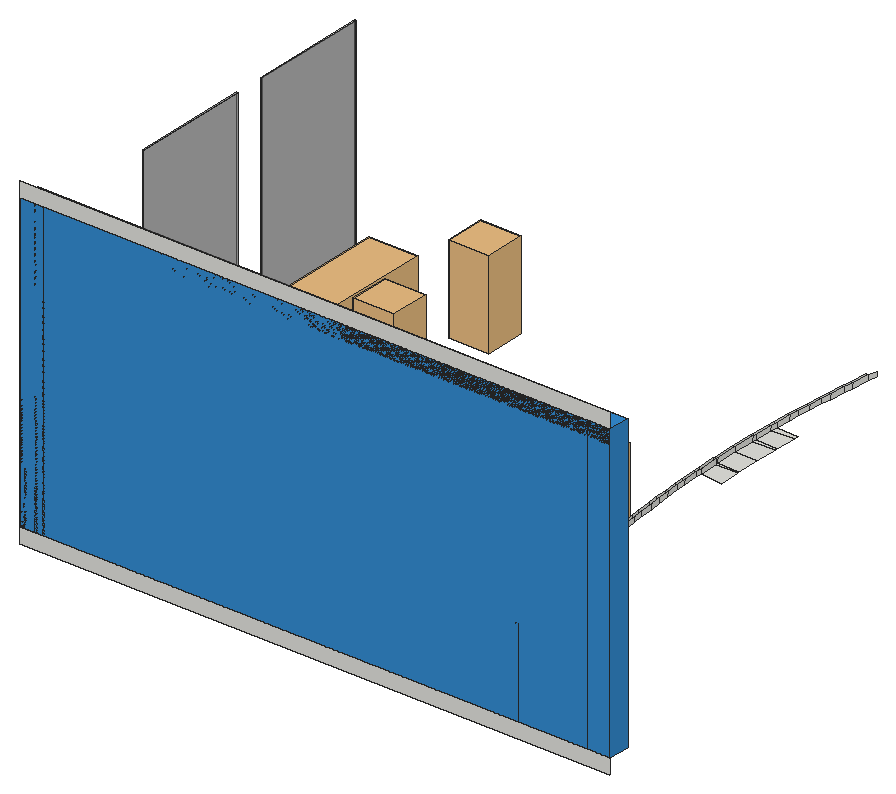
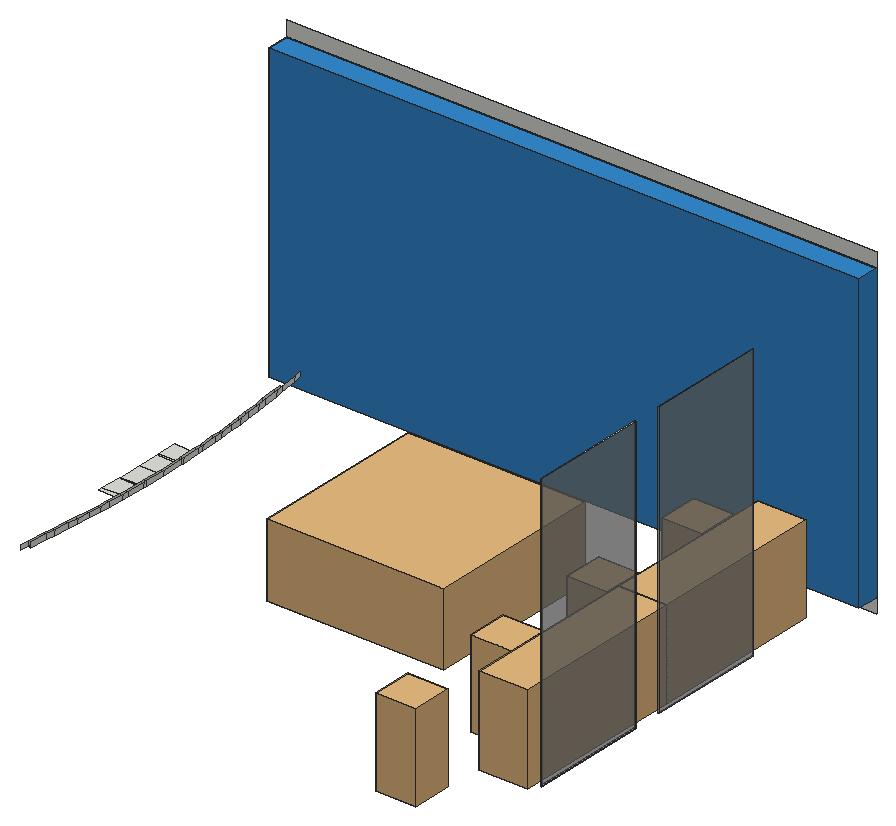
# SketchUp Ruby script. Lengths in inches.
U = 1.inch
M = Sketchup.active_model
def pt(a) = Geom::Point3d.new(a.map { |v| v * U })
def face(e, loops, mat)
  f = e.add_face(loops[0].map { |a| pt(a) })
  loops[1..].each { |l| e.add_face(l.map { |a| pt(a) }).erase! }
  f.material = f.back_material = mat if mat
  f
end
# faces: each face lists its corners as indices into pts; further lists are holes
def faces(e, pts, list, mat = nil) = list.each { |f| face(e, (f[0].is_a?(Array) ? f : [f]).map { |l| l.map { |i| pts[i] } }, mat) }
# xy, xz, yz: faces in a plane at the given z, y or x. An outline is a flat list of corners, or four numbers for a rectangle; further outlines are holes
def ring(l) = l.size == 4 ? [[l[0], l[1]], [l[2], l[1]], [l[2], l[3]], [l[0], l[3]]] : l.each_slice(2).to_a
def flat(e, list, mat, &to3) = list.each { |f| face(e, (f[0].is_a?(Array) ? f : [f]).map { |l| ring(l).map { |u, v| to3.(u, v) } }, mat) }
def xy(e, z, list, mat = nil) = flat(e, list, mat) { |x, y| [x, y, z] }
def xz(e, y, list, mat = nil) = flat(e, list, mat) { |x, z| [x, y, z] }
def yz(e, x, list, mat = nil) = flat(e, list, mat) { |y, z| [x, y, z] }
def lines(e, pts, list) = list.each { |a, b| e.add_line(pt(pts[a]), pt(pts[b])) }
# prism: a flat outline (further loops are holes) pulled along v
def prism(e, loops, v, mat = nil)
  f = face(e, loops, mat); d = Geom::Vector3d.new(v.map { |x| x * U })
  f.pushpull(f.normal.samedirection?(d) ? d.length : -d.length)
end
def box(e, o, s, mat = nil) = prism(e, [[o, [o[0] + s[0], o[1], o[2]], [o[0] + s[0], o[1] + s[1], o[2]], [o[0], o[1] + s[1], o[2]]]], [0, 0, s[2]], mat)
def at(x, y, z, deg = 0) = Geom::Transformation.translation(pt([x, y, z])) * Geom::Transformation.rotation(ORIGIN, Z_AXIS, deg.degrees)
def axes(o, x, y, z) = Geom::Transformation.new([*x, 0, *y, 0, *z, 0, *pt(o).to_a, 1])
def part(name) = M.definitions.add(name)
# library, detail: a bought-in or finely detailed component or shape, given as its bounding box
def library(name, o, s) = part(name).tap { |d| box(d.entities, o, s) }
def detail(e, o, s) = box(e.add_group.entities, o, s)
def put(e, d, t, mat = nil) = e.add_instance(d, t).tap { |i| i.material = mat if mat }
def group(e, t, mat = nil) = e.add_group.tap { |g| g.transformation = t; g.material = mat if mat }.entities
root = M.entities
M.materials.add("[Color I07]").color = [53, 140, 209]
M.materials.add("[Translucent Glass Gray]").color = [128, 128, 128]
M.materials["[Translucent Glass Gray]"].alpha = 0.5
M.materials.add("[Wood Veneer 02]").color = [190, 128, 91]
c1 = library("Edge Console",[-35.43,-9.84,0],[70.86,19.68,29.53])
c2 = library("Group\#15",[-0.03,0,0],[16.43,16.29,39.54])
c3 = library("MARBLE DINING TABLE",[-16.8,-22.21,-0.08],[92.52,94.06,29.61])
c4 = part("Group45\#1")
xz(c4.entities,3.52,[[223.67,42,224.7,44]])
c5 = part("Group49\#1")
xz(c5.entities,3.52,[[21.9,6,30.9,126]],"[Color I07]")
c6 = part("Group53\#1")
xz(c6.entities,3.52,[[21.9,0,261.9,6]])
c7 = part("Group593\#1")
xz(c7.entities,3.52,[[21.9,126.1875,261.9,132.1875]])
c8 = part("Group595\#1")
xz(c8.entities,3.52,[[21.9,120.1875,261.9,126.1875]],"[Color I07]")
c9 = part("Group663\#1")
xz(c9.entities,3.52,[[21.9,6,261.9,126]],"[Color I07]")
c10 = part("Group44\#1")
p = [[252.55,3.52,126],[252.55,3.52,6],[224.7,3.52,42],[224.7,3.52,6],[30.9,3.52,6],[21.9,3.52,6]]
lines(c10.entities,p,[[0,1],[2,3],[4,5]])
put(c10.entities,c4,at(0,0,0))
put(c10.entities,c5,at(0,0,0))
put(c10.entities,c6,at(0,0,0))
put(c10.entities,c7,at(0,0,0))
put(c10.entities,c8,at(0,0,0))
put(c10.entities,c9,at(0,0,0))
c11 = part("Group\#2")
box(c11.entities,[0,0,0],[240,9,120])
xy(root,8,[[4.25,117.22,4.75,165.22]])
xy(root,42,[[191.59,56.57,190.72,64.07,191.71,64.21,192.58,56.72],[190.72,64.07,190.16,67.51,191.15,67.64,191.71,64.21],[190.16,67.51,189.47,74.47,190.46,74.59,191.15,67.64],[189.47,74.47,188.91,78.28,189.91,78.39,190.46,74.59],[188.91,78.28,188.44,84.41,189.43,84.51,189.91,78.39],
  [188.44,84.41,187.87,88.89,188.86,88.98,189.43,84.51],[187.87,88.89,187.59,93.99,188.59,94.0625,188.86,88.98],[187.59,93.99,187.04,99.35,188.04,99.42,188.59,94.0625],[187.04,99.35,186.94,103.28,187.93,103.33,188.04,99.42],[186.94,103.28,186.45,109.7,187.45,109.73,187.93,103.33],
  [186.45,109.7,186.45,112.36,187.45,112.39,187.45,109.73],[196.46,111.52,187.45,112.39,187.1,119.96,196.11,120.15],[186.45,112.36,186.1,119.96,187.1,119.96,187.45,112.39],[186.1,119.96,186.15,121.3125,187.15,121.31,187.1,119.96],[187.1,119.96,187.15,121.31,196.13,120.87,196.11,120.15],
  [196.13,120.87,187.15,121.31,187.01,130.15,196.01,130.15],[187.15,121.31,186.15,121.3125,186.01,130.15,187.01,130.15],[186.01,130.15,186.15,138.99,187.15,139,187.01,130.15],[187.01,130.15,187.15,139,196.13,139.43,196.01,130.15],[186.15,138.99,186.1,140.35,187.1,140.34,187.15,139],
  [187.15,139,187.1,140.34,196.11,140.16,196.13,139.43],[196.11,140.16,187.1,140.34,187.45,147.92,196.46,148.79],[187.1,140.34,186.1,140.35,186.45,147.94,187.45,147.92],[187.45,147.92,186.45,147.94,186.45,150.61,187.45,150.57],[187.45,147.92,187.45,150.57,196.45,150.19,196.46,148.79],
  [187.45,150.57,186.45,150.61,186.94,157.03,187.93,156.98],[187.93,156.98,186.94,157.03,187.04,160.95,188.04,160.89],[188.04,160.89,187.04,160.95,187.59,166.32,188.59,166.24],[188.59,166.24,187.59,166.32,187.87,171.42,188.86,171.33],[188.86,171.33,187.87,171.42,188.44,175.89,189.43,175.79],
  [189.43,175.79,188.44,175.89,188.91,182.03,189.91,181.91],[189.91,181.91,188.91,182.03,189.47,185.83,190.46,185.71],[190.46,185.71,189.47,185.83,190.16,192.8,191.15,192.67]])
xy(root,120,[[4.25,117.22,4.75,165.22]])
xz(root,117.22,[[4.25,8,4.75,120]])
xz(root,165.22,[[4.25,8,4.75,120]])
yz(root,4.25,[[117.22,8,165.22,120]],"[Translucent Glass Gray]")
yz(root,4.75,[[117.22,8,165.22,120]],"[Translucent Glass Gray]")
yz(root,186.45,[[109.7,42,112.36,44],[147.94,42,150.61,44]])
yz(root,187.45,[[109.73,42,112.39,44],[147.92,42,150.57,44]])
p = [[192.21,53.1,44],[191.59,56.57,44],[191.59,56.57,42],[192.21,53.1,42],[190.72,64.07,44],[190.72,64.07,42],
  [190.16,67.51,44],[190.16,67.51,42],[191.71,64.21,44],[191.71,64.21,42],[191.15,67.64,42],[191.15,67.64,44],
  [189.47,74.47,44],[189.47,74.47,42],[190.46,74.59,42],[190.46,74.59,44],[188.91,78.28,44],[188.91,78.28,42],
  [189.91,78.39,42],[189.91,78.39,44],[188.44,84.41,44],[188.44,84.41,42],[189.43,84.51,42],[189.43,84.51,44],
  [187.87,88.89,44],[187.87,88.89,42],[188.86,88.98,42],[188.86,88.98,44],[187.59,93.99,44],[187.59,93.99,42],
  [188.59,94.0625,42],[188.59,94.0625,44],[187.04,99.35,44],[187.04,99.35,42],[188.04,99.42,42],[188.04,99.42,44],
  [186.94,103.28,44],[186.94,103.28,42],[187.93,103.33,42],[187.93,103.33,44],[186.45,109.7,44],[186.45,109.7,42],
  [187.45,109.73,42],[187.45,109.73,44],[186.45,112.36,44],[186.1,119.96,44],[186.1,119.96,42],[186.45,112.36,42],
  [187.45,112.39,44],[187.45,112.39,42],[187.1,119.96,42],[187.1,119.96,44],[186.15,121.3125,44],[186.15,121.3125,42],
  [187.15,121.31,42],[187.15,121.31,44],[186.01,130.15,44],[186.01,130.15,42],[187.01,130.15,42],[187.01,130.15,44],
  [186.15,138.99,44],[186.15,138.99,42],[187.15,139,42],[187.15,139,44],[186.1,140.35,44],[186.1,140.35,42],
  [187.1,140.34,42],[187.1,140.34,44],[186.45,147.94,44],[186.45,147.94,42],[187.45,147.92,42],[187.45,147.92,44],
  [186.45,150.61,44],[186.94,157.03,44],[186.94,157.03,42],[186.45,150.61,42],[187.45,150.57,44],[187.45,150.57,42],
  [187.93,156.98,42],[187.93,156.98,44],[187.04,160.95,44],[187.04,160.95,42],[188.04,160.89,42],[188.04,160.89,44],
  [188.59,166.24,42],[188.59,166.24,44],[187.59,166.32,44],[187.59,166.32,42],[188.86,171.33,42],[188.86,171.33,44],
  [187.87,171.42,44],[187.87,171.42,42],[189.43,175.79,42],[189.43,175.79,44],[188.44,175.89,44],[188.44,175.89,42],
  [189.91,181.91,42],[189.91,181.91,44],[188.91,182.03,44],[188.91,182.03,42],[190.46,185.71,42],[190.46,185.71,44],
  [189.47,185.83,44],[189.47,185.83,42],[191.15,192.67,42],[191.15,192.67,44],[190.16,192.8,44],[190.16,192.8,42],
  [191.71,196.1,42],[191.71,196.1,44]]
faces(root,p,[[0,1,2,3],[1,4,5,2],[4,6,7,5],[8,9,10,11],[6,12,13,7],[11,10,14,15],[12,16,17,13],[15,14,18,19],
  [16,20,21,17],[19,18,22,23],[20,24,25,21],[23,22,26,27],[24,28,29,25],[27,26,30,31],[28,32,33,29],[31,30,34,35],
  [32,36,37,33],[35,34,38,39],[36,40,41,37],[39,38,42,43],[44,45,46,47],[48,49,50,51],[45,52,53,46],[51,50,54,55],
  [52,56,57,53],[55,54,58,59],[56,60,61,57],[59,58,62,63],[60,64,65,61],[63,62,66,67],[64,68,69,65],[67,66,70,71],
  [72,73,74,75],[76,77,78,79],[73,80,81,74],[79,78,82,83],[83,82,84,85],[80,86,87,81],[85,84,88,89],[86,90,91,87],
  [89,88,92,93],[90,94,95,91],[93,92,96,97],[94,98,99,95],[97,96,100,101],[98,102,103,99],[101,100,104,105],[102,106,107,103],
  [105,104,108,109]])
g1 = group(root,at(4.25,57.22,8),"[Translucent Glass Gray]")
box(g1,[0,0,0],[0.5,48,112])
put(root,c1,axes([18.84,130.98,6],[0,1,0],[-1,0,0],[0,0,1.21911]))
put(root,c1,axes([18.84,60.19,6],[0,1,0],[-1,0,0],[0,0,1.21911]),"[Wood Veneer 02]")
put(root,c2,axes([29.5,35.76,6],[1,0,0],[0,1,0],[0,0,0.902]))
put(root,c2,axes([29.5,84.23,6],[1,0,0],[0,1,0],[0,0,0.902]))
put(root,c2,axes([29.5,132.7,6],[1,0,0],[0,1,0],[0,0,0.902]))
put(root,c2,axes([29.5,181.17,6],[1,0,0],[0,1,0],[0,0,0.902]))
put(root,c3,axes([91.21,67.81,6.08],[0.77821,0,0],[0,0.76543,0],[0,0,1]))
put(root,c10,at(-21.9,-3.3,0))
put(root,c11,at(0,0.22,6),"[Color I07]")
